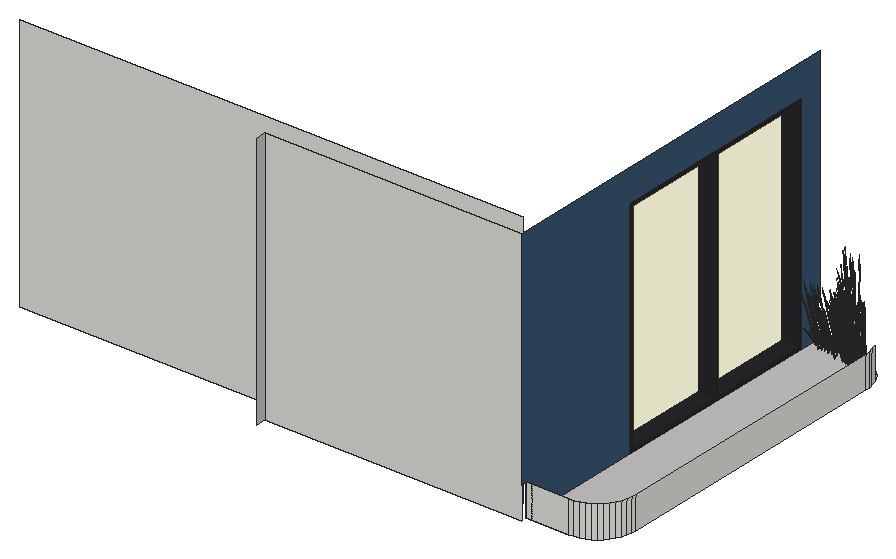
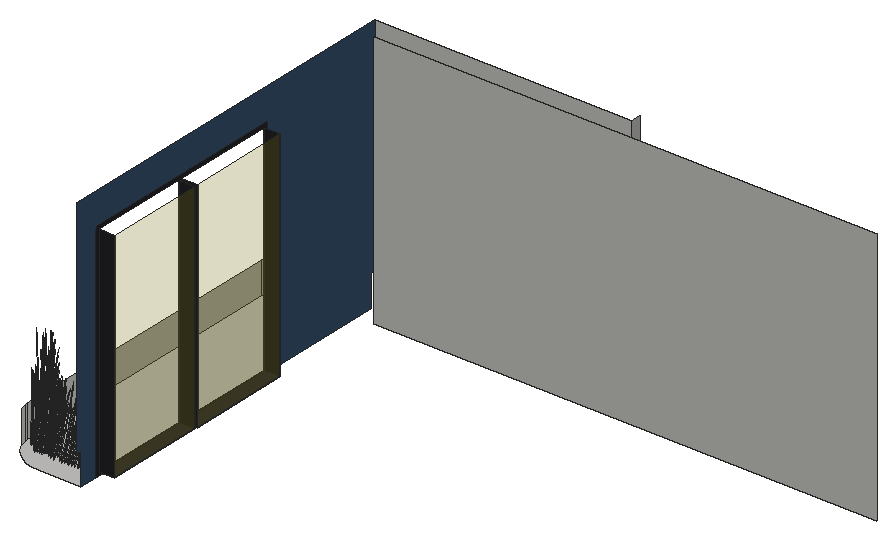
# SketchUp Ruby script. Lengths in inches.
U = 1.inch
M = Sketchup.active_model
def pt(a) = Geom::Point3d.new(a.map { |v| v * U })
def face(e, loops, mat)
  f = e.add_face(loops[0].map { |a| pt(a) })
  loops[1..].each { |l| e.add_face(l.map { |a| pt(a) }).erase! }
  f.material = f.back_material = mat if mat
  f
end
# faces: each face lists its corners as indices into pts; further lists are holes
def faces(e, pts, list, mat = nil) = list.each { |f| face(e, (f[0].is_a?(Array) ? f : [f]).map { |l| l.map { |i| pts[i] } }, mat) }
# xy, xz, yz: faces in a plane at the given z, y or x. An outline is a flat list of corners, or four numbers for a rectangle; further outlines are holes
def ring(l) = l.size == 4 ? [[l[0], l[1]], [l[2], l[1]], [l[2], l[3]], [l[0], l[3]]] : l.each_slice(2).to_a
def flat(e, list, mat, &to3) = list.each { |f| face(e, (f[0].is_a?(Array) ? f : [f]).map { |l| ring(l).map { |u, v| to3.(u, v) } }, mat) }
def xy(e, z, list, mat = nil) = flat(e, list, mat) { |x, y| [x, y, z] }
def xz(e, y, list, mat = nil) = flat(e, list, mat) { |x, z| [x, y, z] }
def yz(e, x, list, mat = nil) = flat(e, list, mat) { |y, z| [x, y, z] }
def lines(e, pts, list) = list.each { |a, b| e.add_line(pt(pts[a]), pt(pts[b])) }
# prism: a flat outline (further loops are holes) pulled along v
def prism(e, loops, v, mat = nil)
  f = face(e, loops, mat); d = Geom::Vector3d.new(v.map { |x| x * U })
  f.pushpull(f.normal.samedirection?(d) ? d.length : -d.length)
end
def box(e, o, s, mat = nil) = prism(e, [[o, [o[0] + s[0], o[1], o[2]], [o[0] + s[0], o[1] + s[1], o[2]], [o[0], o[1] + s[1], o[2]]]], [0, 0, s[2]], mat)
def at(x, y, z, deg = 0) = Geom::Transformation.translation(pt([x, y, z])) * Geom::Transformation.rotation(ORIGIN, Z_AXIS, deg.degrees)
def axes(o, x, y, z) = Geom::Transformation.new([*x, 0, *y, 0, *z, 0, *pt(o).to_a, 1])
def part(name) = M.definitions.add(name)
# library, detail: a bought-in or finely detailed component or shape, given as its bounding box
def library(name, o, s) = part(name).tap { |d| box(d.entities, o, s) }
def detail(e, o, s) = box(e.add_group.entities, o, s)
def put(e, d, t, mat = nil) = e.add_instance(d, t).tap { |i| i.material = mat if mat }
def group(e, t, mat = nil) = e.add_group.tap { |g| g.transformation = t; g.material = mat if mat }.entities
root = M.entities
M.materials.add("Carpet_01_1K").color = [196, 195, 193]
M.materials.add("Carpet_04_1K").color = [56, 85, 112]
M.materials.add("Glass_Basic_01").color = [186, 175, 28]
M.materials["Glass_Basic_01"].alpha = 0.25
M.materials.add("LightPink_Translucent").color = [144, 107, 117]
M.materials["LightPink_Translucent"].alpha = 0.75
M.materials.add("ThomThom - Buttons2").color = [40, 40, 43]
c1 = part("blade")
p = [[2.15,0.21,22],[0,0.17,0],[0.09,0.45,0],[2.18,0.31,22],[2.29,0.31,22],[0.38,0.45,0],
  [2.48,0.24,33],[2.49,0.24,33],[2.48,0.22,33]]
faces(c1.entities,p,[[0,1,2,3],[4,5,2,3],[6,3,4,7],[8,0,3,6]])
c2 = part("seeds")
p = [[0.3,-0.1,1.38],[-0.01,-0.03,1.59],[-0.01,-0.03,0.03],[0.14,-0.07,-0.07],[0.29,-0.03,3],[0.15,0.01,3.11]]
faces(c2.entities,p,[[0,1,2,3],[1,0,4,5]],"LightPink_Translucent")
c3 = part("blade with seeds")
put(c3.entities,c1,at(0,0,0))
put(c3.entities,c2,axes([2.4,0.25,30.99],[1.5799,-0.05474,1.17369],[-0.12525,1.92788,0.29478],[-0.07173,-0.02425,1.56792]))
xy(root,618,[[330.57,158.5,354.57,158.5,357.32,158.68,360.01,159.22,362.61,160.1,365.07,161.31,367.36,162.84,369.42,164.65,371.24,166.72,372.76,169,373.98,171.46,374.86,174.07,375.4,176.76,375.57,179.5,375.57,340.54,375.4,343.28,374.86,345.98,373.98,348.58,372.76,351.04,371.24,353.33,369.42,355.39,367.36,357.2,365.07,358.73,362.61,359.94,360.01,360.83,357.32,361.36,354.57,361.54,330.57,361.54]],"Carpet_01_1K")
xy(root,620,[[321.57,233.15,330.57,291.15],[321.57,293.15,330.57,349.15]],"ThomThom - Buttons2")
xz(root,155.5,[[186.57,618,330.57,762]])
xz(root,158.5,[[330.57,618,333.57,636],[333.57,618,354.57,636]])
xz(root,167.5625,[[39.57,618,321.57,762]])
xz(root,233.15,[[321.57,620,330.57,742]],"ThomThom - Buttons2")
xz(root,291.15,[[321.57,620,330.57,742]],"ThomThom - Buttons2")
xz(root,293.15,[[321.57,620,330.57,742]],"ThomThom - Buttons2")
xz(root,349.15,[[321.57,620,330.57,742]],"ThomThom - Buttons2")
yz(root,186.57,[[149.51,618,155.5,762]],"Carpet_01_1K")
yz(root,321.57,[[233.15,620,291.15,742],[293.15,620,349.15,742]],"Glass_Basic_01")
yz(root,330.57,[[158.5,618,231.15,618,231.15,744,351.15,744,351.15,618,361.54,618,361.54,636,364.54,636,364.54,762,155.5,762,155.5,636,158.5,636]],"Carpet_04_1K")
yz(root,330.57,[[[231.15,618,351.15,744],[233.15,620,233.15,742,349.15,742,349.15,620,293.15,620,293.15,742,291.15,742,291.15,620]]],"ThomThom - Buttons2")
yz(root,375.57,[[179.5,618,340.54,636]])
p = [[357.32,158.68,618],[354.57,158.5,618],[354.57,158.5,636],[357.32,158.68,636],[360.01,159.22,618],[360.01,159.22,636],
  [362.61,160.1,618],[362.61,160.1,636],[365.07,161.31,618],[365.07,161.31,636],[367.36,162.84,618],[367.36,162.84,636],
  [369.42,164.65,618],[369.42,164.65,636],[371.24,166.72,618],[371.24,166.72,636],[372.76,169,618],[372.76,169,636],
  [373.98,171.46,618],[373.98,171.46,636],[374.86,174.07,618],[374.86,174.07,636],[375.4,176.76,618],[375.4,176.76,636],
  [375.57,179.5,618],[375.57,179.5,636],[375.4,343.28,618],[375.57,340.54,618],[375.57,340.54,636],[375.4,343.28,636],
  [374.86,345.98,618],[374.86,345.98,636],[373.98,348.58,618],[373.98,348.58,636]]
faces(root,p,[[0,1,2,3],[4,0,3,5],[6,4,5,7],[8,6,7,9],[10,8,9,11],[12,10,11,13],[14,12,13,15],[16,14,15,17],
  [18,16,17,19],[20,18,19,21],[22,20,21,23],[24,22,23,25],[26,27,28,29],[30,26,29,31],[32,30,31,33]])
put(root,c3,axes([359.82,349.34,621.875],[0.08068,0.14973,1.71376],[-0.3728,0.12606,0.13857],[-0.08426,-0.23506,0.73262]))
put(root,c3,axes([360.44,348.34,622.72],[-0.05398,-0.06539,1.74944],[-0.36026,0.04145,-0.27667],[-0.0575,-0.15639,0.14031]))
put(root,c3,axes([361.28,349.12,620.59],[-0.10032,0.0944,1.43002],[-0.30046,-0.16522,-0.30754],[0.05569,-0.20547,0.61141]))
put(root,c3,axes([360.82,349.45,622.98],[-0.16845,-0.3792,-0.71045],[0.34676,-0.21133,0.08574],[-0.03939,-0.18322,1.00501]))
put(root,c3,axes([359.72,348.94,620.59],[-0.02137,0.15256,1.43002],[-0.31245,0.12771,-0.30754],[-0.07303,-0.19719,0.61141]))
put(root,c3,axes([360.53,348.61,619.49],[-0.0592,0.0168,1.76342],[-0.32738,-0.18913,-0.26939],[0.00549,-0.15776,0.30037]))
put(root,c3,axes([361.52,349.82,622.98],[0.00918,-0.43138,-0.71045],[0.38672,0.02897,0.08574],[0.04081,-0.18275,1.00501]))
put(root,c3,axes([362.06,349.15,622.72],[-0.00341,-0.09282,1.74944],[-0.28775,-0.26825,-0.27667],[0.04449,-0.16261,0.14031]))
put(root,c3,axes([360.85,349.13,622.53],[0.1064,-0.35863,-0.35414],[0.31043,0.1046,0.4572],[-0.02846,-0.14439,0.87481]))
put(root,c3,axes([361.08,349.6,621.875],[-0.06572,0.16029,1.71376],[-0.27569,-0.33172,0.13857],[0.12437,-0.20675,0.73262]))
put(root,c3,axes([361.98,348.8125,622.71],[-0.03584,0.03562,1.77383],[-0.35118,-0.12018,-0.16761],[-0.01271,-0.15545,0.31391]))
put(root,c3,axes([360.69,349.37,622.68],[-0.34695,-0.11691,-0.51099],[0.11892,-0.40083,-0.3958],[-0.03181,-0.16138,0.97773]))
put(root,c3,axes([360.91,348.37,620.77],[0.04528,0.27194,1.1486],[-0.25117,-0.15062,0.84392],[0.02703,-0.13924,0.25299]))
put(root,c3,axes([361.44,349.68,622.68],[-0.25266,-0.31335,-0.51099],[0.2669,-0.27442,-0.3958],[0.03844,-0.15921,0.97773]))
put(root,c3,axes([360.07,348.13,622.71],[-0.00658,0.0559,1.77383],[-0.32474,0.20287,-0.16761],[-0.09556,-0.1037,0.31391]))
put(root,c3,axes([360,349.12,623.09],[0.39316,-0.11987,0.53763],[0.06823,0.47021,0.4433],[-0.09247,-0.13858,1.11249]))
put(root,c3,axes([360.89,349.21,622.73],[0.34777,0.12192,0.48003],[-0.11892,0.40083,0.3958],[-0.0209,-0.15763,0.9933]))
put(root,c3,axes([360.99,349.35,623.03],[-0.34538,0.21713,-0.1216],[-0.16972,-0.38536,-0.67495],[-0.04557,-0.16239,1.02557]))
put(root,c3,axes([361.71,349.84,623.03],[-0.3879,-0.02311,-0.1216],[0.0106,-0.43749,-0.67495],[0.02694,-0.1685,1.02557]))
put(root,c3,axes([361.68,349.5625,622.53],[0.23881,-0.24554,-0.35414],[0.22606,0.28036,0.4572],[0.0344,-0.14245,0.87481]))
put(root,c3,axes([359.61,348.7,620.77],[0.18411,0.16231,1.1486],[-0.26813,0.09757,0.84392],[-0.05737,-0.12474,0.25299]))
put(root,c3,axes([360.98,349.18,622.73],[0.26007,-0.1585,0.0643],[0.12729,0.28902,0.50621],[-0.02512,-0.1274,0.77189]))
put(root,c3,axes([360.06,349.56,622.98],[-0.30095,-0.22541,-0.71045],[0.21388,-0.395,0.08574],[-0.10904,-0.13459,1.00501]))
put(root,c3,axes([359.95,349.26,622.53],[-0.05451,-0.37564,-0.35414],[0.31161,-0.09919,0.4572],[-0.0837,-0.10765,0.87481]))
put(root,c3,axes([360.09,349.22,622.73],[0.16041,-0.29625,0.0643],[0.22843,0.17248,0.50621],[-0.07385,-0.09498,0.77189]))
put(root,c3,axes([359.47,349.1875,619.49],[-0.03419,0.06144,1.76342],[-0.3455,0.13246,-0.26939],[-0.08346,-0.12049,0.30037]))
put(root,c3,axes([363.44,351.19,621.875],[0.08068,0.14973,1.71376],[-0.3728,0.12606,0.13857],[-0.08426,-0.23506,0.73262]))
put(root,c3,axes([360.04,350.875,620.1],[-0.14494,-0.47823,-0.69835],[0.41752,-0.17223,-0.18329],[-0.01602,-0.16194,1.54149]))
put(root,c3,axes([359.28,349.8,621.875],[0.1311,0.08035,1.71376],[-0.27131,0.33708,0.13857],[-0.16909,-0.15206,0.73262]))
put(root,c3,axes([361.98,349.41,619.49],[-0.05283,-0.03674,1.76342],[-0.13569,-0.41045,-0.26939],[0.09154,-0.11138,0.30037]))
put(root,c3,axes([364.06,350.2,622.72],[-0.05398,-0.06539,1.74944],[-0.36026,0.04145,-0.27667],[-0.0575,-0.15639,0.14031]))
put(root,c3,axes([364.89,350.97,620.59],[-0.10032,0.0944,1.43002],[-0.30046,-0.16522,-0.30754],[0.05569,-0.20547,0.61141]))
put(root,c3,axes([360.88,349.5,623.05],[-0.1064,0.35863,0.35414],[-0.31043,-0.1046,-0.4572],[-0.02846,-0.14439,0.87481]))
put(root,c3,axes([364.43,351.3,622.98],[-0.16845,-0.3792,-0.71045],[0.34676,-0.21133,0.08574],[-0.03939,-0.18322,1.00501]))
put(root,c3,axes([359.92,349.57,622.68],[-0.34827,0.11086,-0.51099],[-0.06092,-0.41983,-0.3958],[-0.09354,-0.12031,0.97773]))
put(root,c3,axes([361.68,349.66,622.73],[0.25132,0.3182,0.48003],[-0.2669,0.27442,0.3958],[0.04636,-0.14929,0.9933]))
put(root,c3,axes([363.34,350.8,620.59],[-0.02137,0.15256,1.43002],[-0.31245,0.12771,-0.30754],[-0.07303,-0.19719,0.61141]))
put(root,c3,axes([360.16,349.19,623.43],[-0.23555,0.44708,-0.13619],[-0.34112,-0.25757,-0.75594],[-0.11858,-0.12631,1.14864]))
put(root,c3,axes([361.77,349.6875,622.73],[0.29004,0.02173,0.0643],[-0.00795,0.32812,0.50621],[0.03035,-0.12569,0.77189]))
put(root,c3,axes([364.14,350.46,619.49],[-0.0592,0.0168,1.76342],[-0.32738,-0.18913,-0.26939],[0.00549,-0.15776,0.30037]))
put(root,c3,axes([361.55,349.91,623.05],[-0.23881,0.24554,0.35414],[-0.22606,-0.28036,-0.4572],[0.0344,-0.14245,0.87481]))
put(root,c3,axes([361.97,350.57,622.98],[0.18436,-0.36797,-0.71045],[0.32306,0.26151,0.08574],[0.11008,-0.13332,1.00501]))
put(root,c3,axes([359.98,349.5,620.375],[-0.22066,-0.46731,0],[0.36918,-0.26061,-0.51607],[0.08408,-0.05936,1.63711]))
put(root,c3,axes([361.97,350.4,622.68],[-0.09067,-0.42583,-0.51099],[0.34336,-0.07449,-0.3958],[0.0984,-0.11438,0.97773]))
put(root,c3,axes([365.13,351.67,622.98],[0.00918,-0.43138,-0.71045],[0.38672,0.02897,0.08574],[0.04081,-0.18275,1.00501]))
put(root,c3,axes([360.47,348.9375,620.13],[-0.2439,0.26754,-0.03893],[-0.22348,-0.29302,-0.17649],[-0.01573,-0.08303,0.58215]))
put(root,c3,axes([365.67,351,622.72],[-0.00341,-0.09282,1.74944],[-0.28775,-0.26825,-0.27667],[0.04449,-0.16261,0.14031]))
put(root,c3,axes([364.47,350.98,622.53],[0.1064,-0.35863,-0.35414],[0.31043,0.1046,0.4572],[-0.02846,-0.14439,0.87481]))
put(root,c3,axes([364.7,351.45,621.875],[-0.06572,0.16029,1.71376],[-0.27569,-0.33172,0.13857],[0.12437,-0.20675,0.73262]))
put(root,c3,axes([365.6,350.67,622.71],[-0.03584,0.03562,1.77383],[-0.35118,-0.12018,-0.16761],[-0.01271,-0.15545,0.31391]))
put(root,c3,axes([359.26,349.06,622.72],[-0.07594,-0.00329,1.74944],[-0.24177,0.32918,-0.27667],[-0.129,-0.06726,0.14031]))
put(root,c3,axes([362.13,350.7,623.03],[-0.32648,-0.25715,-0.1216],[0.18809,-0.3724,-0.67495],[0.09224,-0.12945,1.02557]))
put(root,c3,axes([364.31,351.23,622.68],[-0.34695,-0.11691,-0.51099],[0.11892,-0.40083,-0.3958],[-0.03181,-0.16138,0.97773]))
put(root,c3,axes([364.52,350.22,620.77],[0.04528,0.27194,1.1486],[-0.25117,-0.15062,0.84392],[0.02703,-0.13924,0.25299]))
put(root,c3,axes([360.78,352.11,621.33],[0.305,0.18805,1.51261],[-0.29879,0.40513,0.59816],[-0.13384,-0.24012,1.26806]))
put(root,c3,axes([365.06,351.53,622.68],[-0.25266,-0.31335,-0.51099],[0.2669,-0.27442,-0.3958],[0.03844,-0.15921,0.97773]))
put(root,c3,axes([360.14,349.56,623.05],[0.05451,0.37564,0.35414],[-0.31161,0.09919,-0.4572],[-0.0837,-0.10765,0.87481]))
put(root,c3,axes([359.18,350.81,620.02],[0,-0.46636,-0.49651],[0.39487,0,0],[0,-0.10622,1.57504]))
put(root,c3,axes([360.28,349.43,620.02],[0.33032,-0.23318,-0.49651],[0.19744,0.41812,0],[0.07523,-0.05311,1.57504]))
put(root,c3,axes([363.6875,349.98,622.71],[-0.00658,0.0559,1.77383],[-0.32474,0.20287,-0.16761],[-0.09556,-0.1037,0.31391]))
put(root,c3,axes([362.24,350.23,620.59],[-0.12609,-0.01381,1.43002],[-0.12917,-0.37055,-0.30754],[0.1549,-0.10482,0.61141]))
put(root,c3,axes([359.2,349.81,623.09],[0.29147,-0.34417,0.53763],[0.25138,0.3655,0.4433],[-0.13675,-0.06349,1.11249]))
put(root,c3,axes([362.93,350.59,622.71],[-0.0461,-0.00354,1.77383],[-0.19143,-0.37951,-0.16761],[0.07688,-0.12478,0.31391]))
put(root,c3,axes([360.67,350.38,620.06],[0.23773,-0.35053,-0.62353],[0.29532,0.31785,-0.16365],[0.09526,-0.08744,1.37633]))
put(root,c3,axes([362.39,349.55,620.77],[-0.11756,0.2374,1.1486],[-0.10105,-0.31895,0.84392],[0.09709,-0.07992,0.25299]))
put(root,c3,axes([363.61,350.98,623.09],[0.39316,-0.11987,0.53763],[0.06823,0.47021,0.4433],[-0.09247,-0.13858,1.11249]))
put(root,c3,axes([364.5,351.0625,622.73],[0.34777,0.12192,0.48003],[-0.11892,0.40083,0.3958],[-0.0209,-0.15763,0.9933]))
put(root,c3,axes([354.95,352.49,621.875],[0.08068,0.14973,1.71376],[-0.3728,0.12606,0.13857],[-0.08426,-0.23506,0.73262]))
put(root,c3,axes([364.6,351.21,623.03],[-0.34538,0.21713,-0.1216],[-0.16972,-0.38536,-0.67495],[-0.04557,-0.16239,1.02557]))
put(root,c3,axes([365.32,351.69,623.03],[-0.3879,-0.02311,-0.1216],[0.0106,-0.43749,-0.67495],[0.02694,-0.1685,1.02557]))
put(root,c3,axes([365.29,351.41,622.53],[0.23881,-0.24554,-0.35414],[0.22606,0.28036,0.4572],[0.0344,-0.14245,0.87481]))
put(root,c3,axes([363.23,350.55,620.77],[0.18411,0.16231,1.1486],[-0.26813,0.09757,0.84392],[-0.05737,-0.12474,0.25299]))
put(root,c3,axes([364.6,351.03,622.73],[0.26007,-0.1585,0.0643],[0.12729,0.28902,0.50621],[-0.02512,-0.1274,0.77189]))
put(root,c3,axes([363.67,351.41,622.98],[-0.30095,-0.22541,-0.71045],[0.21388,-0.395,0.08574],[-0.10904,-0.13459,1.00501]))
put(root,c3,axes([362.22,350.44,622.53],[0.30722,-0.06665,-0.35414],[0.08112,0.381,0.4572],[0.08804,-0.10234,0.87481]))
put(root,c3,axes([355.5625,351.5,622.72],[-0.05398,-0.06539,1.74944],[-0.36026,0.04145,-0.27667],[-0.0575,-0.15639,0.14031]))
put(root,c3,axes([363.57,351.11,622.53],[-0.05451,-0.37564,-0.35414],[0.31161,-0.09919,0.4572],[-0.0837,-0.10765,0.87481]))
put(root,c3,axes([359.34,349.81,622.73],[0.01777,-0.35463,0.0643],[0.26836,0.00972,0.50621],[-0.1028,-0.03711,0.77189]))
put(root,c3,axes([356.4,352.27,620.59],[-0.10032,0.0944,1.43002],[-0.30046,-0.16522,-0.30754],[0.05569,-0.20547,0.61141]))
put(root,c3,axes([360.26,351,620.21],[0.17124,-0.42022,-0.44739],[0.35581,0.20224,0.21531],[0,-0.09687,1.43643]))
put(root,c3,axes([359.23,349.92,622.53],[-0.20082,-0.29199,-0.35414],[0.2293,-0.2764,0.4572],[-0.1165,-0.04206,0.87481]))
put(root,c3,axes([355.94,352.6,622.98],[-0.16845,-0.3792,-0.71045],[0.34676,-0.21133,0.08574],[-0.03939,-0.18322,1.00501]))
put(root,c3,axes([360.42,350.79,620.67],[-0.04113,-0.53214,-0.29095],[0.42835,-0.03218,-0.50002],[0.07543,-0.07088,1.59708]))
put(root,c3,axes([352.79,352.76,621.875],[0.08068,0.14973,1.71376],[-0.3728,0.12606,0.13857],[-0.08426,-0.23506,0.73262]))
put(root,c3,axes([359.35,350.82,620.03],[0.24637,-0.29097,-0.30978],[0.24637,0.29097,0.30978],[0,-0.09372,1.38974]))
put(root,c3,axes([354.84,352.1,620.59],[-0.02137,0.15256,1.43002],[-0.31245,0.12771,-0.30754],[-0.07303,-0.19719,0.61141]))
put(root,c3,axes([359.25,349.42,620.13],[-0.10181,0.3808,-0.03893],[-0.31336,-0.11714,-0.17649],[-0.04758,-0.06228,0.58215]))
put(root,c3,axes([361.97,350.67,623.05],[-0.30722,0.06665,0.35414],[-0.08112,-0.381,-0.4572],[0.08804,-0.10234,0.87481]))
put(root,c3,axes([360.22,351.35,620.67],[-0.39748,-0.22252,-0.29095],[0.19139,-0.46966,-0.50002],[-0.01249,-0.11531,1.59708]))
put(root,c3,axes([353.41,351.77,622.72],[-0.05398,-0.06539,1.74944],[-0.36026,0.04145,-0.27667],[-0.0575,-0.15639,0.14031]))
put(root,c3,axes([355.65,351.76,619.49],[-0.0592,0.0168,1.76342],[-0.32738,-0.18913,-0.26939],[0.00549,-0.15776,0.30037]))
put(root,c3,axes([359.09,351.16,620.375],[-0.44133,0,0],[0,-0.52122,-0.51607],[0,-0.11871,1.63711]))
put(root,c3,axes([354.24,352.55,620.59],[-0.10032,0.0944,1.43002],[-0.30046,-0.16522,-0.30754],[0.05569,-0.20547,0.61141]))
put(root,c3,axes([359.16,350.23,620.59],[0.06891,0.12984,1.43002],[-0.15879,0.35293,-0.30754],[-0.16304,-0.08436,0.61141]))
put(root,c3,axes([363.7,351.08,622.73],[0.16041,-0.29625,0.0643],[0.22843,0.17248,0.50621],[-0.07385,-0.09498,0.77189]))
put(root,c3,axes([353.78,352.875,622.98],[-0.16845,-0.3792,-0.71045],[0.34676,-0.21133,0.08574],[-0.03939,-0.18322,1.00501]))
put(root,c3,axes([363.08,351.04,619.49],[-0.03419,0.06144,1.76342],[-0.3455,0.13246,-0.26939],[-0.08346,-0.12049,0.30037]))
put(root,c3,axes([348.2,353,621.875],[0.08068,0.14973,1.71376],[-0.3728,0.12606,0.13857],[-0.08426,-0.23506,0.73262]))
put(root,c3,axes([360.36,349.61,620.03],[0.32928,0.11539,-0.30978],[-0.08291,0.40636,0.30978],[0.06638,-0.04686,1.38974]))
put(root,c3,axes([352.6875,352.37,620.59],[-0.02137,0.15256,1.43002],[-0.31245,0.12771,-0.30754],[-0.07303,-0.19719,0.61141]))
put(root,c3,axes([356.64,352.97,622.98],[0.00918,-0.43138,-0.71045],[0.38672,0.02897,0.08574],[0.04081,-0.18275,1.00501]))
put(root,c3,axes([363.65,352.73,620.1],[-0.14494,-0.47823,-0.69835],[0.41752,-0.17223,-0.18329],[-0.01602,-0.16194,1.54149]))
put(root,c3,axes([348.8125,352.01,622.72],[-0.05398,-0.06539,1.74944],[-0.36026,0.04145,-0.27667],[-0.0575,-0.15639,0.14031]))
put(root,c3,axes([362.9,351.66,621.875],[0.1311,0.08035,1.71376],[-0.27131,0.33708,0.13857],[-0.16909,-0.15206,0.73262]))
put(root,c3,axes([359.45,350.11,622.98],[-0.35281,-0.01123,-0.71045],[0.0237,-0.47284,0.08574],[-0.14947,-0.0499,1.00501]))
put(root,c3,axes([365.59,351.27,619.49],[-0.05283,-0.03674,1.76342],[-0.13569,-0.41045,-0.26939],[0.09154,-0.11138,0.30037]))
put(root,c3,axes([353.49,352.04,619.49],[-0.0592,0.0168,1.76342],[-0.32738,-0.18913,-0.26939],[0.00549,-0.15776,0.30037]))
put(root,c3,axes([349.65,352.78,620.59],[-0.10032,0.0944,1.43002],[-0.30046,-0.16522,-0.30754],[0.05569,-0.20547,0.61141]))
put(root,c3,axes([357.18,352.3,622.72],[-0.00341,-0.09282,1.74944],[-0.28775,-0.26825,-0.27667],[0.04449,-0.16261,0.14031]))
put(root,c3,axes([355.97,352.28,622.53],[0.1064,-0.35863,-0.35414],[0.31043,0.1046,0.4572],[-0.02846,-0.14439,0.87481]))
put(root,c3,axes([356.21,352.75,621.875],[-0.06572,0.16029,1.71376],[-0.27569,-0.33172,0.13857],[0.12437,-0.20675,0.73262]))
put(root,c3,axes([357.1,351.97,622.71],[-0.03584,0.03562,1.77383],[-0.35118,-0.12018,-0.16761],[-0.01271,-0.15545,0.31391]))
put(root,c3,axes([349.19,353.11,622.98],[-0.16845,-0.3792,-0.71045],[0.34676,-0.21133,0.08574],[-0.03939,-0.18322,1.00501]))
put(root,c3,axes([341.22,353.24,621.875],[0.08068,0.14973,1.71376],[-0.3728,0.12606,0.13857],[-0.08426,-0.23506,0.73262]))
put(root,c3,axes([345.13,353.25,621.875],[0.08068,0.14973,1.71376],[-0.3728,0.12606,0.13857],[-0.08426,-0.23506,0.73262]))
put(root,c3,axes([364.5,351.36,623.05],[-0.1064,0.35863,0.35414],[-0.31043,-0.1046,-0.4572],[-0.02846,-0.14439,0.87481]))
put(root,c3,axes([348.09,352.6,620.59],[-0.02137,0.15256,1.43002],[-0.31245,0.12771,-0.30754],[-0.07303,-0.19719,0.61141]))
put(root,c3,axes([337.54,353.32,621.875],[0.08068,0.14973,1.71376],[-0.3728,0.12606,0.13857],[-0.08426,-0.23506,0.73262]))
put(root,c3,axes([362.25,350.61,622.73],[0.2423,0.19613,0.0643],[-0.14107,0.2793,0.50621],[0.07768,-0.0903,0.77189]))
put(root,c3,axes([363.53,351.42,622.68],[-0.34827,0.11086,-0.51099],[-0.06092,-0.41983,-0.3958],[-0.09354,-0.12031,0.97773]))
put(root,c3,axes([354.48,353.25,622.98],[0.00918,-0.43138,-0.71045],[0.38672,0.02897,0.08574],[0.04081,-0.18275,1.00501]))
put(root,c3,axes([365.29,351.51,622.73],[0.25132,0.3182,0.48003],[-0.2669,0.27442,0.3958],[0.04636,-0.14929,0.9933]))
put(root,c3,axes([343.09,353.34,621.875],[0.08068,0.14973,1.71376],[-0.3728,0.12606,0.13857],[-0.08426,-0.23506,0.73262]))
put(root,c3,axes([341.83,352.25,622.72],[-0.05398,-0.06539,1.74944],[-0.36026,0.04145,-0.27667],[-0.0575,-0.15639,0.14031]))
put(root,c3,axes([362.18,350.53,622.73],[0.08753,0.42921,0.48003],[-0.34336,0.07449,0.3958],[0.1012,-0.10094,0.9933]))
put(root,c3,axes([345.75,352.26,622.72],[-0.05398,-0.06539,1.74944],[-0.36026,0.04145,-0.27667],[-0.0575,-0.15639,0.14031]))
put(root,c3,axes([363.78,351.05,623.43],[-0.23555,0.44708,-0.13619],[-0.34112,-0.25757,-0.75594],[-0.11858,-0.12631,1.14864]))
put(root,c3,axes([355.8125,352.53,622.68],[-0.34695,-0.11691,-0.51099],[0.11892,-0.40083,-0.3958],[-0.03181,-0.16138,0.97773]))
put(root,c3,axes([363.11,351.04,622.72],[0.04898,-0.07104,1.74944],[-0.06269,-0.43574,-0.27667],[0.12289,-0.08262,0.14031]))
put(root,c3,axes([356.03,351.52,620.77],[0.04528,0.27194,1.1486],[-0.25117,-0.15062,0.84392],[0.02703,-0.13924,0.25299]))
put(root,c3,axes([365.39,351.54,622.73],[0.29004,0.02173,0.0643],[-0.00795,0.32812,0.50621],[0.03035,-0.12569,0.77189]))
put(root,c3,axes([357.77,353.39,621.875],[0.08068,0.14973,1.71376],[-0.3728,0.12606,0.13857],[-0.08426,-0.23506,0.73262]))
put(root,c3,axes([359.3,353.41,621.875],[0.08068,0.14973,1.71376],[-0.3728,0.12606,0.13857],[-0.08426,-0.23506,0.73262]))
put(root,c3,axes([348.9,352.27,619.49],[-0.0592,0.0168,1.76342],[-0.32738,-0.18913,-0.26939],[0.00549,-0.15776,0.30037]))
put(root,c3,axes([342.67,353.02,620.59],[-0.10032,0.0944,1.43002],[-0.30046,-0.16522,-0.30754],[0.05569,-0.20547,0.61141]))
put(root,c3,axes([338.15,352.32,622.72],[-0.05398,-0.06539,1.74944],[-0.36026,0.04145,-0.27667],[-0.0575,-0.15639,0.14031]))
put(root,c3,axes([346.58,353.03,620.59],[-0.10032,0.0944,1.43002],[-0.30046,-0.16522,-0.30754],[0.05569,-0.20547,0.61141]))
put(root,c3,axes([343.7,352.35,622.72],[-0.05398,-0.06539,1.74944],[-0.36026,0.04145,-0.27667],[-0.0575,-0.15639,0.14031]))
put(root,c3,axes([356.5625,352.83,622.68],[-0.25266,-0.31335,-0.51099],[0.2669,-0.27442,-0.3958],[0.03844,-0.15921,0.97773]))
put(root,c3,axes([355.02,352.57,622.72],[-0.00341,-0.09282,1.74944],[-0.28775,-0.26825,-0.27667],[0.04449,-0.16261,0.14031]))
put(root,c3,axes([342.21,353.35,622.98],[-0.16845,-0.3792,-0.71045],[0.34676,-0.21133,0.08574],[-0.03939,-0.18322,1.00501]))
put(root,c3,axes([353.82,352.55,622.53],[0.1064,-0.35863,-0.35414],[0.31043,0.1046,0.4572],[-0.02846,-0.14439,0.87481]))
put(root,c3,axes([354.05,353.03,621.875],[-0.06572,0.16029,1.71376],[-0.27569,-0.33172,0.13857],[0.12437,-0.20675,0.73262]))
put(root,c3,axes([354.95,352.24,622.71],[-0.03584,0.03562,1.77383],[-0.35118,-0.12018,-0.16761],[-0.01271,-0.15545,0.31391]))
put(root,c3,axes([346.125,353.36,622.98],[-0.16845,-0.3792,-0.71045],[0.34676,-0.21133,0.08574],[-0.03939,-0.18322,1.00501]))
put(root,c3,axes([365.17,351.76,623.05],[-0.23881,0.24554,0.35414],[-0.22606,-0.28036,-0.4572],[0.0344,-0.14245,0.87481]))
put(root,c3,axes([338.99,353.1,620.59],[-0.10032,0.0944,1.43002],[-0.30046,-0.16522,-0.30754],[0.05569,-0.20547,0.61141]))
put(root,c3,axes([358.38,352.4,622.72],[-0.05398,-0.06539,1.74944],[-0.36026,0.04145,-0.27667],[-0.0575,-0.15639,0.14031]))
put(root,c3,axes([359.43,351.02,620.33],[-0.32829,0.39208,0.30756],[-0.32849,-0.38796,-0.36492],[-0.01146,-0.11134,1.64885]))
put(root,c3,axes([359.92,352.41,622.72],[-0.05398,-0.06539,1.74944],[-0.36026,0.04145,-0.27667],[-0.0575,-0.15639,0.14031]))
put(root,c3,axes([344.54,353.12,620.59],[-0.10032,0.0944,1.43002],[-0.30046,-0.16522,-0.30754],[0.05569,-0.20547,0.61141]))
put(root,c3,axes([341.11,352.84,620.59],[-0.02137,0.15256,1.43002],[-0.31245,0.12771,-0.30754],[-0.07303,-0.19719,0.61141]))
put(root,c3,axes([338.53,353.43,622.98],[-0.16845,-0.3792,-0.71045],[0.34676,-0.21133,0.08574],[-0.03939,-0.18322,1.00501]))
put(root,c3,axes([355.19,351.28,622.71],[-0.00658,0.0559,1.77383],[-0.32474,0.20287,-0.16761],[-0.09556,-0.1037,0.31391]))
put(root,c3,axes([345.03,352.85,620.59],[-0.02137,0.15256,1.43002],[-0.31245,0.12771,-0.30754],[-0.07303,-0.19719,0.61141]))
put(root,c3,axes([365.59,352.42,622.98],[0.18436,-0.36797,-0.71045],[0.32306,0.26151,0.08574],[0.11008,-0.13332,1.00501]))
put(root,c3,axes([344.08,353.45,622.98],[-0.16845,-0.3792,-0.71045],[0.34676,-0.21133,0.08574],[-0.03939,-0.18322,1.00501]))
put(root,c3,axes([363.6,351.35,620.375],[-0.22066,-0.46731,0],[0.36918,-0.26061,-0.51607],[0.08408,-0.05936,1.63711]))
put(root,c3,axes([365.58,352.25,622.68],[-0.09067,-0.42583,-0.51099],[0.34336,-0.07449,-0.3958],[0.0984,-0.11438,0.97773]))
put(root,c3,axes([358.97,349.34,622.71],[0.02617,0.04654,1.77383],[-0.12614,0.41836,-0.16761],[-0.12775,0.00303,0.31391]))
put(root,c3,axes([349.89,353.48,622.98],[0.00918,-0.43138,-0.71045],[0.38672,0.02897,0.08574],[0.04081,-0.18275,1.00501]))
put(root,c3,axes([359.22,353.18,620.59],[-0.10032,0.0944,1.43002],[-0.30046,-0.16522,-0.30754],[0.05569,-0.20547,0.61141]))
put(root,c3,axes([360.75,353.1875,620.59],[-0.10032,0.0944,1.43002],[-0.30046,-0.16522,-0.30754],[0.05569,-0.20547,0.61141]))
